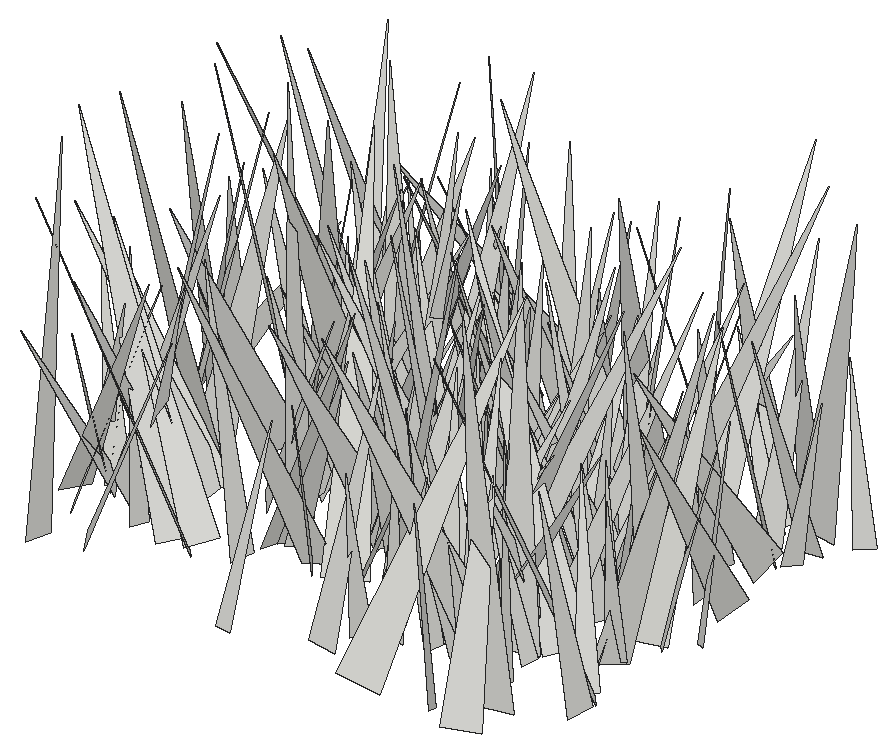
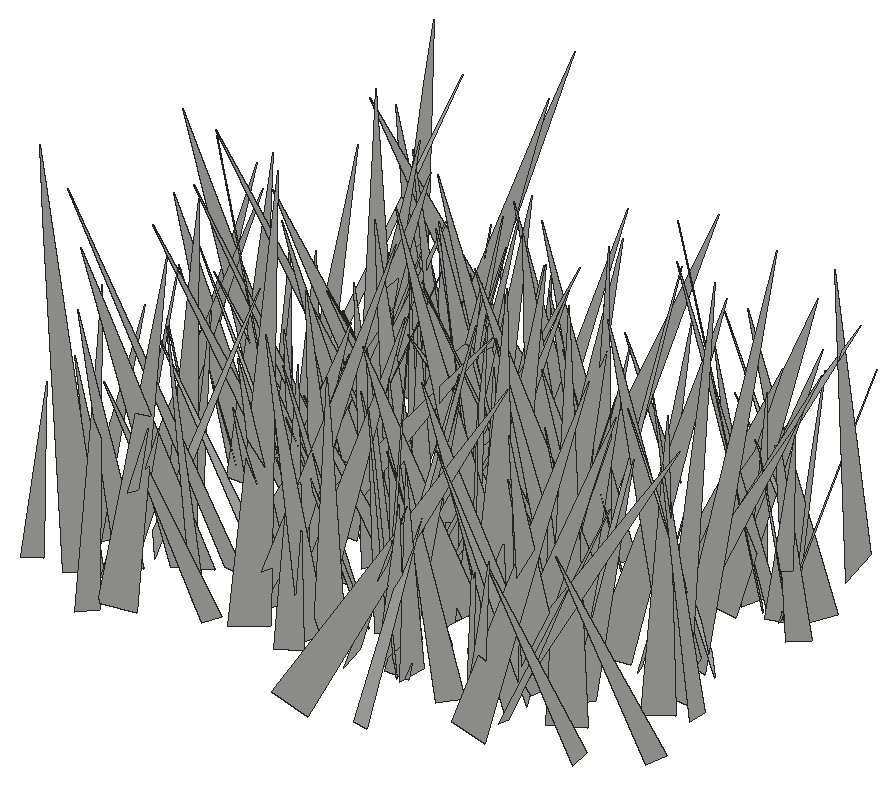
# SketchUp Ruby script. Lengths in inches.
U = 1.inch
M = Sketchup.active_model
def pt(a) = Geom::Point3d.new(a.map { |v| v * U })
def face(e, loops, mat)
  f = e.add_face(loops[0].map { |a| pt(a) })
  loops[1..].each { |l| e.add_face(l.map { |a| pt(a) }).erase! }
  f.material = f.back_material = mat if mat
  f
end
# faces: each face lists its corners as indices into pts; further lists are holes
def faces(e, pts, list, mat = nil) = list.each { |f| face(e, (f[0].is_a?(Array) ? f : [f]).map { |l| l.map { |i| pts[i] } }, mat) }
# xy, xz, yz: faces in a plane at the given z, y or x. An outline is a flat list of corners, or four numbers for a rectangle; further outlines are holes
def ring(l) = l.size == 4 ? [[l[0], l[1]], [l[2], l[1]], [l[2], l[3]], [l[0], l[3]]] : l.each_slice(2).to_a
def flat(e, list, mat, &to3) = list.each { |f| face(e, (f[0].is_a?(Array) ? f : [f]).map { |l| ring(l).map { |u, v| to3.(u, v) } }, mat) }
def xy(e, z, list, mat = nil) = flat(e, list, mat) { |x, y| [x, y, z] }
def xz(e, y, list, mat = nil) = flat(e, list, mat) { |x, z| [x, y, z] }
def yz(e, x, list, mat = nil) = flat(e, list, mat) { |y, z| [x, y, z] }
def lines(e, pts, list) = list.each { |a, b| e.add_line(pt(pts[a]), pt(pts[b])) }
# prism: a flat outline (further loops are holes) pulled along v
def prism(e, loops, v, mat = nil)
  f = face(e, loops, mat); d = Geom::Vector3d.new(v.map { |x| x * U })
  f.pushpull(f.normal.samedirection?(d) ? d.length : -d.length)
end
def box(e, o, s, mat = nil) = prism(e, [[o, [o[0] + s[0], o[1], o[2]], [o[0] + s[0], o[1] + s[1], o[2]], [o[0], o[1] + s[1], o[2]]]], [0, 0, s[2]], mat)
def at(x, y, z, deg = 0) = Geom::Transformation.translation(pt([x, y, z])) * Geom::Transformation.rotation(ORIGIN, Z_AXIS, deg.degrees)
def axes(o, x, y, z) = Geom::Transformation.new([*x, 0, *y, 0, *z, 0, *pt(o).to_a, 1])
def part(name) = M.definitions.add(name)
# library, detail: a bought-in or finely detailed component or shape, given as its bounding box
def library(name, o, s) = part(name).tap { |d| box(d.entities, o, s) }
def detail(e, o, s) = box(e.add_group.entities, o, s)
def put(e, d, t, mat = nil) = e.add_instance(d, t).tap { |i| i.material = mat if mat }
def group(e, t, mat = nil) = e.add_group.tap { |g| g.transformation = t; g.material = mat if mat }.entities
root = M.entities
c1 = part("fur_instance\#9")
p = [[0.8125,0,1.79],[0.67,-0.02,1.48],[0,-0.11,0],[0,0.11,0]]
faces(c1.entities,p,[[0,1,2,3]])
put(root,c1,axes([111.79,435.77,-27.1],[-2.18486,3.79279,1.02862],[3.92891,2.13324,0.47945],[0.08359,-1.13179,4.35074]))
put(root,c1,axes([111.93,431,-27.1],[-7.13651,-0.0123,2.39844],[-0.61978,7.28244,-1.80677],[2.31701,1.91008,6.90402]))
put(root,c1,axes([108.84,446.41,-27.1],[1.93678,-3.59499,0.72466],[-3.24209,-1.29543,2.2385],[1.71404,1.61186,3.41529]))
put(root,c1,axes([109.68,443.03,-27.1],[5.83398,1.13984,1.03884],[1.35175,-5.73614,-1.2974],[-0.74243,-1.48703,5.80098]))
put(root,c1,axes([111.72,435.73,-27.1],[-3.93384,-2.91751,0.42121],[-2.51987,3.69278,2.04402],[1.52955,-1.41982,4.45073]))
put(root,c1,axes([111.57,435.41,-27.1],[-2.88957,-1.62735,2.00469],[-2.2228,3.09866,-0.68855],[1.31385,1.66334,3.24403]))
put(root,c1,axes([110.3,436.45,-27.1],[2.04033,-4.0488,0.48109],[-4.03745,-1.93127,0.8697],[0.56854,0.81522,4.44965]))
put(root,c1,axes([110.85,443.78,-27.1],[3.52243,-4.25283,0.7835],[-4.27225,-3.57882,-0.21878],[-0.66956,0.46198,5.5178]))
put(root,c1,axes([112.21,440.22,-27.1],[-2.39726,-7.68863,1.50052],[-7.81274,2.46126,0.12966],[0.5725,1.39306,8.05265]))
put(root,c1,axes([111.07,442.56,-27.1],[-1.7083,-7.51191,1.45388],[-7.48357,1.95063,1.28533],[1.59333,1.10775,7.59572]))
put(root,c1,axes([111.57,439.72,-27.1],[4.49985,4.45709,1.03745],[4.28289,-4.6143,1.2473],[-1.61209,0.1822,6.20956]))
put(root,c1,axes([111.3,435.7,-27.1],[-2.16154,-4.08693,0.6496],[-3.73051,2.24163,1.68984],[1.79115,-0.26331,4.30345]))
put(root,c1,axes([114.72,437.71,-27.1],[-4.43376,3.47486,0.22998],[3.34427,4.14468,1.85019],[-0.97128,-1.59146,5.32068]))
put(root,c1,axes([114.79,437.59,-27.1],[-6.1435,0.43905,0.01492],[0.43419,6.03663,1.1429],[-0.06685,-1.14104,6.05221]))
put(root,c1,axes([116.16,446.22,-27.1],[-4.67528,-5.85921,0.505],[-5.43274,4.05599,-3.23694],[-2.25181,2.37953,6.76097]))
put(root,c1,axes([111.5,433.51,-27.1],[4.04394,2.43918,0.42992],[2.39305,-4.06014,0.52577],[-0.63852,0.23141,4.69325]))
put(root,c1,axes([115.94,434.08,-27.1],[-4.22364,6.9226,0.63988],[6.72709,3.88063,2.42031],[-1.75445,-1.78585,7.73974]))
put(root,c1,axes([111.04,448.03,-27.1],[4.1398,0.29454,0.02134],[0.28882,-4.10074,0.57065],[-0.06159,0.56772,4.11084]))
put(root,c1,axes([110.67,434.7,-27.1],[5.28357,-2.5058,0.04843],[-2.504,-5.27298,0.35108],[0.10676,0.33794,5.83712]))
put(root,c1,axes([113.52,444.75,-27.1],[-4.62696,1.13691,1.70574],[1.48296,4.76376,0.84751],[1.41525,-1.27471,4.68861]))
put(root,c1,axes([113.81,436.46,-27.1],[0.77993,-5.26102,0.56712],[-5.12867,-0.89269,-1.22806],[-1.30258,0.36472,5.1748]))
put(root,c1,axes([114.15,433.99,-27.1],[-5.02502,0.15502,0.9974],[-0.08895,4.97687,-1.22169],[1.00545,1.21508,4.87671]))
put(root,c1,axes([113.43,441.62,-27.1],[-3.15969,-2.10838,0.70871],[-1.88389,3.19122,1.09464],[1.18257,-0.54957,3.6374]))
put(root,c1,axes([116.91,433.47,-27.1],[-5.49378,-4.48735,0.1731],[-4.21573,5.05933,-2.64174],[-1.54724,2.14821,6.58325]))
put(root,c1,axes([116.55,444.95,-27.1],[-3.06653,-6.21678,2.70439],[-6.51984,1.89062,-3.04678],[-1.85842,3.62531,6.22648]))
put(root,c1,axes([112.43,440.375,-27.1],[-0.87926,6.56228,2.62812],[6.83144,1.46959,-1.38397],[1.81713,-2.34956,6.47466]))
put(root,c1,axes([114.84,447.625,-27.1],[-4.29176,-1.39668,0.34406],[-1.22552,4.11722,1.42648],[0.75311,-1.25938,4.28195]))
put(root,c1,axes([115.32,449.05,-27.1],[-0.75565,-7.24529,1.23648],[-7.25287,0.53359,-1.30585],[-1.19119,1.34729,7.16659]))
put(root,c1,axes([116.74,434.33,-27.1],[-3.94655,4.7323,0.06828],[4.56087,3.77904,1.70056],[-1.26405,-1.13963,5.92267]))
put(root,c1,axes([115.15,444.92,-27.1],[-6.13848,3.83375,0.83292],[3.60337,6.1212,-1.61832],[1.55148,0.95163,7.05405]))
put(root,c1,axes([112.15,435.48,-27.1],[3.4737,5.90005,1.74495],[6.11319,-3.08303,-1.74525],[0.69596,-2.36778,6.62052]))
put(root,c1,axes([113.13,435.06,-27.1],[5.7382,5.20942,1.87337],[5.41352,-5.84467,-0.3291],[-1.15821,-1.50876,7.74318]))
put(root,c1,axes([113.33,435.24,-27.1],[4.73571,-1.08461,0.9225],[-1.0987,-4.82145,-0.02851],[-0.90568,0.17765,4.85824]))
put(root,c1,axes([114.72,441.66,-27.1],[4.75153,-4.99406,0.9078],[-4.47168,-4.70683,-2.48828],[-2.40183,-1.11663,6.42854]))
put(root,c1,axes([112.9,446.44,-27.1],[1.80193,-7.44469,0.50754],[-7.36471,-1.69029,1.35351],[1.20089,0.80465,7.53912]))
put(root,c1,axes([116.74,440.5,-27.1],[-6.42891,-4.93695,1.78859],[-5.18873,6.40682,-0.96596],[0.80598,1.86616,8.04806]))
put(root,c1,axes([116.12,447.69,-27.1],[0.1057,3.9764,0.92499],[3.9126,-0.36287,1.11284],[-1.16573,-0.85739,3.81897]))
put(root,c1,axes([113.4,431.88,-27.1],[4.3525,2.53578,0.43229],[2.57081,-4.2585,-0.90411],[0.08934,-0.99816,4.9555]))
put(root,c1,axes([115.09,442.33,-27.1],[4.32331,2.64676,1.47041],[2.57631,-4.56233,0.63737],[-1.59061,-0.19566,5.02892]))
put(root,c1,axes([116.06,443.05,-27.1],[-2.49672,2.92464,0.96124],[2.97957,2.60694,-0.1927],[0.77439,-0.6012,3.84057]))
put(root,c1,axes([115.46,445.33,-27.1],[5.32876,3.34285,1.26399],[2.90072,-5.37113,1.97605],[-2.08763,1.0697,5.97207]))
put(root,c1,axes([116.81,442.59,-27.1],[-4.46885,1.59045,1.08144],[1.18804,4.43404,-1.61169],[1.51249,1.21632,4.46123]))
put(root,c1,axes([115.78,444.75,-27.1],[5.60712,-6.07402,0.33398],[-5.83929,-5.5015,-2.02021],[-1.70529,-1.13347,8.01575]))
put(root,c1,axes([114.31,443.875,-27.1],[6.51578,-0.90085,0.09034],[-0.89347,-6.50413,-0.41604],[-0.1463,-0.39981,6.56459]))
put(root,c1,axes([117.02,443.31,-27.1],[-4.18199,-2.55213,0.91155],[-1.98836,4.02848,2.15666],[1.84139,-1.44616,4.39901]))
put(root,c1,axes([118.53,434.42,-27.1],[-5.56537,0.35389,1.01892],[0.25962,5.63719,-0.53984],[1.04691,0.48332,5.55042]))
put(root,c1,axes([118.64,437.53,-27.1],[-8.04005,-0.21045,2.18635],[-0.63833,8.16213,-1.56173],[2.10165,1.67397,7.88972]))
put(root,c1,axes([117.86,439.8125,-27.1],[-4.50462,1.14541,2.32905],[1.86637,4.67145,1.31236],[1.80364,-1.97324,4.45884]))
put(root,c1,axes([116.33,444.74,-27.1],[-3.15581,4.82371,2.67558],[4.59437,4.00448,-1.80054],[3.05265,-1.04019,5.47589]))
put(root,c1,axes([118.45,443.82,-27.1],[5.58768,-4.04107,3.86555],[-4.58295,-6.44048,-0.10822],[-3.20457,2.16447,6.89498]))
put(root,c1,axes([116.71,447.23,-27.1],[-2.8265,-4.26887,1.57231],[-3.66111,3.23328,2.19698],[2.70032,-0.08465,4.62446]))
put(root,c1,axes([117.77,444.52,-27.1],[1.5026,-5.2869,1.47769],[-5.48951,-1.44343,0.41772],[0.01326,1.53554,5.48039]))
put(root,c1,axes([116.67,438.11,-27.1],[3.8282,2.91024,0.83789],[3.01788,-3.55309,-1.44728],[0.25298,-1.65308,4.58585]))
put(root,c1,axes([116.37,440.34,-27.1],[6.24865,-3.61776,1.18124],[-3.80474,-5.99015,1.78079],[-0.08657,2.13519,6.99733]))
put(root,c1,axes([118.68,451,-27.1],[-3.43446,-5.67079,0.15135],[-5.3482,3.29577,2.1239],[1.89143,-0.97791,6.28032]))
put(root,c1,axes([119.51,447.02,-27.1],[-4.59387,1.36569,1.34916],[1.20913,4.77619,-0.71765],[1.49109,0.33451,4.73854]))
put(root,c1,axes([117.33,447.59,-27.1],[2.31038,-4.41979,0.71264],[-4.3801,-2.06578,1.38834],[0.92579,1.25629,4.79008]))
put(root,c1,axes([120.58,446.91,-27.1],[-3.8761,2.85036,0.12124],[2.83481,3.87102,-0.37744],[0.32105,0.23257,4.79648]))
put(root,c1,axes([121.63,451.375,-27.1],[2.28844,-6.77562,0.58153],[-5.77223,-2.2597,-3.61376],[-3.59563,-0.68473,6.17144]))
put(root,c1,axes([120.97,435.77,-27.1],[0.32689,-6.93131,1.01824],[-6.72809,-0.59471,-1.88835],[-1.95261,0.88881,6.67713]))
put(root,c1,axes([119.48,436.3,-27.1],[4.39596,-0.31282,2.17467],[-1.10489,-4.51925,1.5834],[-1.89902,1.90528,4.11281]))
put(root,c1,axes([120.54,441,-27.1],[-3.35147,5.54659,2.9979],[6.27053,3.28643,0.92965],[0.65767,-3.06906,6.41348]))
put(root,c1,axes([121.12,446.57,-27.1],[-6.29577,-3.22015,2.48262],[-3.79064,6.30377,-1.43636],[1.47099,2.46225,6.92409]))
put(root,c1,axes([121.97,447.4,-27.1],[-4.83845,-0.36416,0.05457],[-0.36621,4.6838,-1.21411],[-0.03844,1.21473,4.69778]))
put(root,c1,axes([119.9375,447.37,-27.1],[-0.22883,-5.12281,0.23524],[-5.12454,0.23734,0.18366],[0.19416,0.22665,5.12463]))
put(root,c1,axes([120.32,447.08,-27.1],[3.4021,4.35261,1.87369],[4.47593,-3.70904,0.48912],[-1.55627,-1.15238,5.50275]))
put(root,c1,axes([117.35,440.14,-27.1],[4.17015,5.48726,0.52169],[5.30168,-3.81404,-2.26221],[1.50809,-1.76505,6.51019]))
put(root,c1,axes([120.72,442.78,-27.1],[-6.29891,4.40553,1.36932],[3.82289,6.28157,-2.62437],[2.58248,1.44677,7.22479]))
put(root,c1,axes([118.68,440.96,-27.1],[2.58495,3.56171,0.23056],[3.43761,-2.40789,-1.34382],[0.96012,-0.96809,4.1907]))
put(root,c1,axes([119.54,440.2,-27.1],[4.26328,-1.39926,0.74192],[-1.39292,-4.32659,-0.15583],[-0.75375,0.08115,4.48433]))
put(root,c1,axes([119.57,444.69,-27.1],[3.16954,2.48643,0.53995],[2.54162,-3.13416,-0.48689],[-0.1185,-0.71733,3.99891]))
put(root,c1,axes([120.68,442.48,-27.1],[5.22033,-0.21574,2.13038],[0.1303,-5.5713,-0.88347],[-2.13731,-0.86658,5.14955]))
put(root,c1,axes([122.38,435.47,-27.1],[-3.14428,7.71271,0.49149],[7.72648,3.12546,0.38342],[-0.17032,-0.59964,8.32018]))
put(root,c1,axes([122.85,439.9,-27.1],[-6.22259,1.31552,1.1088],[1.51746,6.15727,1.21077],[0.81078,-1.42761,6.24382]))
put(root,c1,axes([119.25,436.41,-27.1],[4.36325,-2.68491,0.18726],[-2.69098,-4.34538,0.39756],[0.04948,0.43666,5.1077]))
put(root,c1,axes([121.28,429.87,-27.1],[1.03899,3.82207,0.22987],[3.79032,-1.06041,0.49963],[-0.54276,-0.08876,3.92914]))
put(root,c1,axes([118.87,436.01,-27.1],[6.16535,-1.94029,0.16764],[-1.94054,-6.16752,-0.01601],[-0.16472,0.03505,6.46343]))
put(root,c1,axes([122.63,443.95,-27.1],[-6.25427,-0.78477,1.30734],[-0.71032,6.38344,0.43371],[1.34924,-0.27711,6.28838]))
put(root,c1,axes([118.12,443.25,-27.1],[8.10386,-2.02713,0.06413],[-2.02706,-8.10412,-0.01624],[-0.06615,-0.00019,8.35354]))
put(root,c1,axes([120.83,435.52,-27.1],[-2.98653,-2.99705,1.42564],[-2.58075,3.30304,1.53746],[2.08674,-0.20437,3.94181]))
put(root,c1,axes([121.02,438.68,-27.1],[4.46685,2.95329,0.59597],[2.75098,-4.43263,1.34675],[-1.2285,0.81223,5.18275]))
put(root,c1,axes([121.8,438.78,-27.1],[6.11084,-2.63091,1.80363],[-1.49433,-5.80472,-3.40432],[-2.81811,-2.62692,5.71618]))
put(root,c1,axes([121.27,445.14,-27.1],[3.01124,-3.84874,1.35887],[-4.04465,-3.04041,0.35153],[-0.54781,1.29229,4.87409]))
put(root,c1,axes([124.53,439.91,-27.1],[-6.85321,0.30824,0.48855],[0.41589,6.6696,1.62593],[0.40091,-1.64973,6.66467]))
put(root,c1,axes([123.75,440.92,-27.1],[-4.70083,-1.74871,0.0814],[-1.70109,4.61801,0.97093],[0.41342,-0.88228,4.92068]))
put(root,c1,axes([123.51,446.72,-27.1],[-0.65155,5.99766,1.58433],[6.18323,0.49957,0.65163],[-0.49968,-1.63861,5.99765]))
put(root,c1,axes([122.21,438.33,-27.1],[6.62959,-1.41825,2.66639],[-1.99694,-6.88369,1.30369],[-2.26567,1.91728,6.65307]))
put(root,c1,axes([122.86,438.14,-27.1],[2.86729,-4.50295,0.62999],[-4.43501,-2.93396,-0.78577],[-1.00209,0.10064,5.2802]))
put(root,c1,axes([122.16,440.4375,-27.1],[1.97582,-3.11414,0.08334],[-3.10691,-1.9626,0.3224],[0.22782,0.24287,3.67393]))
put(root,c1,axes([124.13,436.48,-27.1],[-7.73799,2.57835,1.8542],[1.9672,7.72518,-2.53263],[2.4932,1.90688,7.75308]))
put(root,c1,axes([125.91,437.43,-27.1],[-7.81157,-0.92448,1.21309],[-1.13809,7.74743,-1.42443],[1.01538,1.5715,7.73604]))
put(root,c1,axes([124.1,437.6875,-27.1],[1.75802,-6.33898,1.96931],[-6.51413,-2.03906,-0.74828],[-1.27556,1.67662,6.53555]))
put(root,c1,axes([123.1,435.31,-27.1],[4.98815,3.01806,0.37753],[2.59556,-4.60182,2.49383],[-1.58564,1.9615,5.26983]))
put(root,c1,axes([122.125,445.13,-27.1],[0.90872,-5.0896,0.45336],[-4.90772,-0.74115,1.51668],[1.42262,0.69427,4.94262]))
put(root,c1,axes([124.6,446.9375,-27.1],[2.95346,-5.37759,1.21149],[-5.08452,-3.18852,-1.75785],[-2.12927,0.1548,5.87804]))
put(root,c1,axes([128.625,441.75,-27.1],[-5.00631,-5.98003,0.73957],[-5.22244,3.82659,-4.41068],[-3.00563,3.31169,6.43193]))
put(root,c1,axes([126.08,437.46,-27.1],[-6.2227,2.39174,0.32304],[2.36421,6.22042,-0.51348],[0.48507,0.36431,6.64671]))
put(root,c1,axes([126.85,446.18,-27.1],[-8.04315,1.60644,1.39343],[1.83623,7.99603,1.38066],[1.07265,-1.64234,8.08496]))
put(root,c1,axes([123.91,442.05,-27.1],[3.88682,0.49651,1.01606],[0.42112,-4.01087,0.34905],[-1.04955,0.22945,3.90283]))
put(root,c1,axes([123.05,445.28,-27.1],[2.48404,3.35431,0.63876],[3.34518,-2.23213,-1.28736],[0.685,-1.26336,3.97047]))
put(root,c1,axes([127.67,435.57,-27.1],[-6.96753,-1.64469,0.65915],[-1.76863,6.61713,-2.18437],[0.10697,2.27915,6.81763]))
put(root,c1,axes([125.1875,443.42,-27.1],[1.99951,5.4557,0.6063],[5.41529,-2.06607,0.73224],[-0.89823,-0.31139,5.76424]))
put(root,c1,axes([123.96,447.08,-27.1],[5.74343,-0.59024,1.12729],[-0.57342,-5.85294,-0.14303],[-1.13593,-0.02976,5.77191]))
put(root,c1,axes([123.78,442.05,-27.1],[-0.24087,4.17753,0.95098],[3.88217,0.61574,-1.72155],[1.81241,-0.76371,3.81393]))
put(root,c1,axes([124.8,431.11,-27.1],[0.44242,5.64748,1.29703],[5.78226,-0.34572,-0.46699],[0.37666,-1.32609,5.6455]))
put(root,c1,axes([124.14,448.28,-27.1],[1.58205,-4.94043,0.08132],[-4.90313,-1.55912,0.66773],[0.6114,0.28046,5.1444]))
put(root,c1,axes([125.51,434,-27.1],[-5.11664,3.91829,0.85035],[3.38571,4.96082,-2.48663],[2.14782,1.51438,5.94556]))
put(root,c1,axes([125.46,432.53,-27.1],[2.03457,-2.99845,1.01926],[-3.06758,-2.16697,-0.25148],[-0.78708,0.69471,3.61482]))
put(root,c1,axes([124.48,440.99,-27.1],[4.31409,-4.88001,1.43702],[-5.06352,-4.30068,0.59646],[-0.49016,1.47666,6.48614]))
put(root,c1,axes([125.49,441.46,-27.1],[-4.36102,2.95909,2.58691],[3.11538,4.95832,-0.41976],[2.39639,-1.06094,5.25343]))
put(root,c1,axes([128.03,433.61,-27.1],[-6.43885,-0.2283,0.73687],[-0.34147,6.39798,-1.00159],[0.69173,1.03328,6.36457]))
put(root,c1,axes([123.48,439.1875,-27.1],[7.4678,0.08394,0.57516],[0.2355,-7.21321,-2.00499],[-0.53141,-2.01703,7.1941]))
put(root,c1,axes([126.61,437.625,-27.1],[-4.17339,1.81444,1.20525],[1.74242,4.34394,-0.50613],[1.30721,0.0026,4.52253]))
put(root,c1,axes([126.13,432.95,-27.1],[6.62272,2.03005,2.53711],[1.31072,-6.93962,2.13125],[-2.97322,1.46257,6.59085]))
put(root,c1,axes([124.73,439.93,-27.1],[0.74077,3.76285,1.03817],[3.63302,-0.27816,-1.5841],[1.42759,-1.24465,3.49262]))
put(root,c1,axes([126.15,443.51,-27.1],[-1.18817,5.57554,2.26119],[5.96275,1.39894,-0.31626],[0.80332,-2.13721,5.69196]))
put(root,c1,axes([126.49,433.08,-27.1],[0.16475,-3.83195,1.51207],[-4.1166,-0.0965,0.20397],[0.15418,1.51796,3.83006]))
put(root,c1,axes([129.53,438.83,-27.1],[-6.43064,-2.17008,0.24743],[-2.17262,6.27662,-1.4168],[-0.22404,1.42068,6.6374]))
put(root,c1,axes([126.78,440.1,-27.1],[2.27684,-3.73592,1.683],[-3.94498,-2.51908,-0.25488],[-1.10756,1.29258,4.36763]))
put(root,c1,axes([129.45,433.69,-27.1],[-0.93338,-7.69941,2.7531],[-7.87622,0.10215,-2.38461],[-2.19672,2.90522,7.38009]))
put(root,c1,axes([126.33,432.98,-27.1],[2.59266,-2.6088,0.97622],[-2.78019,-2.50569,0.68761],[-0.17141,1.18171,3.61316]))
put(root,c1,axes([126.36,445.94,-27.1],[-1.839,3.01934,1.93742],[3.07994,2.44517,-0.88715],[1.83955,-1.07548,3.42218]))
put(root,c1,axes([128.46,444,-27.1],[-4.34148,-1.68145,0.56308],[-1.64517,4.37512,0.38015],[0.66161,-0.1544,4.64018]))
put(root,c1,axes([128.1,434.09,-27.1],[-0.91047,5.0165,1.03079],[5.11456,0.83694,0.44447],[-0.2628,-1.09133,5.07905]))
put(root,c1,axes([127.39,437.1,-27.1],[4.14484,0.5886,1.74948],[0.68446,-4.48393,-0.11303],[-1.71425,-0.36717,4.1849]))
put(root,c1,axes([128.9,443.1875,-27.1],[0.42359,6.38348,0.10104],[6.1795,-0.43539,1.60081],[-1.60398,0.00839,6.194]))
put(root,c1,axes([126.3,447.83,-27.1],[7.64117,-3.1953,0.94942],[-2.87226,-7.51641,-2.18001],[-1.69158,-1.67105,7.9903]))
put(root,c1,axes([125.59,437.76,-27.1],[2.92691,3.10527,0.26779],[2.82947,-2.4932,-2.01476],[1.3071,-1.55642,3.76168]))
put(root,c1,axes([128.03,440.64,-27.1],[0.49777,-7.47829,0.86543],[-7.52286,-0.52678,-0.22508],[-0.28353,0.84808,7.49146]))
put(root,c1,axes([129.28,434.875,-27.1],[-7.73279,0.49202,2.83462],[1.75633,7.24586,3.53356],[2.27869,-3.91518,6.89581]))
put(root,c1,axes([130.17,441.54,-27.1],[0.21984,-5.04241,1.33274],[-4.72838,-0.75562,-2.0789],[-2.20101,1.11963,4.59917]))
put(root,c1,axes([126.64,436.78,-27.1],[0.2906,4.64928,0.9365],[4.41539,0.07727,-1.75374],[1.73123,-0.9775,4.31562]))
put(root,c1,axes([130.64,438.02,-27.1],[-3.35511,-5.27651,0.83113],[-5.27558,3.11951,-1.49198],[-0.83701,1.48869,6.07225]))
put(root,c1,axes([128.56,440.55,-27.1],[-0.5351,4.97369,0.08314],[4.96853,0.53845,-0.2337],[0.24128,-0.05757,4.99693]))
put(root,c1,axes([127.36,439.38,-27.1],[0.34617,6.42334,1.62872],[6.51894,-0.03728,-1.2385],[1.18972,-1.66468,6.31231]))
put(root,c1,axes([131.8125,436.34,-27.1],[-7.18183,4.15456,0.03319],[4.14203,7.15453,0.70461],[-0.3242,-0.62648,8.26695]))
put(root,c1,axes([131.4,438.75,-27.1],[0.1109,6.16383,0.84068],[5.38265,-0.51661,3.07768],[-3.11876,-0.67243,5.34163]))
put(root,c1,axes([130.74,430.02,-27.1],[-5.03149,-1.83162,1.20846],[-2.18082,4.50919,-2.24552],[0.24343,2.5384,4.86091]))
put(root,c1,axes([129.83,440.49,-27.1],[-3.46593,0.7925,0.89611],[1.04093,3.35143,1.06213],[0.58952,-1.25841,3.39303]))
put(root,c1,axes([128.09,437.3125,-27.1],[4.34491,0.59069,1.09524],[0.90101,-4.23706,-1.28924],[-0.85828,-1.45776,4.19106]))
put(root,c1,axes([127.49,429.8125,-27.1],[-1.94232,7.80928,1.11049],[7.41359,2.19794,-2.48968],[2.69386,-0.41817,7.65238]))
put(root,c1,axes([129.58,446.77,-27.1],[-5.36603,-1.88935,2.74168],[-2.67241,5.54565,-1.40882],[1.98613,2.35731,5.51173]))
put(root,c1,axes([129.06,441.46,-27.1],[0.06663,3.86387,1.64805],[4.18879,0.06273,-0.31643],[0.31563,-1.6482,3.85147]))
put(root,c1,axes([128.0625,436.15,-27.1],[6.72656,-0.08852,1.07497],[-0.40385,-6.50233,1.99163],[-1.00015,2.03024,6.42556]))
put(root,c1,axes([131.33,434.8125,-27.1],[-3.91396,0.19988,0.40503],[0.19284,3.93443,-0.07818],[0.40843,0.05784,3.91828]))
put(root,c1,axes([127.61,448.34,-27.1],[1.13497,4.33314,1.68645],[4.04549,-0.06445,-2.557],[2.29221,-2.03177,3.67778]))
put(root,c1,axes([130.5,435.17,-27.1],[1.64686,-6.77743,3.62945],[-7.62252,-1.92308,-0.13234],[-1.0018,3.49096,6.97339]))
put(root,c1,axes([132.68,445.33,-27.1],[-5.08452,-4.09315,0.88657],[-4.17476,4.84247,-1.58557],[-0.33349,1.78573,6.33184]))
put(root,c1,axes([131.56,433.22,-27.1],[-4.31752,-0.25034,0.73123],[-0.52227,4.00392,-1.71296],[0.56974,1.77322,3.97108]))
put(root,c1,axes([130.98,436.93,-27.1],[-4.32918,-1.79601,0.73607],[-1.48596,4.22424,1.56749],[1.24875,-1.19977,4.41706]))
put(root,c1,axes([128.19,436.72,-27.1],[3.14457,7.68443,0.45621],[7.56933,-2.99688,-1.69436],[1.40136,-1.05601,8.12822]))
put(root,c1,axes([130.8125,449.74,-27.1],[2.01145,-6.31603,1.30369],[-6.40118,-2.12156,-0.40211],[-0.78536,1.11557,6.61638]))
put(root,c1,axes([132.23,448.24,-27.1],[-2.23276,3.13779,0.67741],[3.20125,2.1153,0.75324],[-0.23799,-0.9847,3.77672]))
put(root,c1,axes([130.43,442.67,-27.1],[4.1336,3.03674,0.5342],[2.87698,-4.11997,1.15876],[-1.10914,0.6308,4.99657]))
put(root,c1,axes([132.42,447.4,-27.1],[-3.36159,2.04077,0.19725],[2.04893,3.35754,0.1809],[0.07444,-0.25709,3.9284]))
put(root,c1,axes([130.5,445.8125,-27.1],[-1.86477,7.56726,1.18834],[7.49142,2.05683,-1.34204],[1.5982,-0.81177,7.67722]))
put(root,c1,axes([128.96,435.21,-27.1],[4.72114,-1.50275,0.05764],[-1.46013,-4.53503,1.361],[0.36002,1.31378,4.76394]))
put(root,c1,axes([131.54,430.97,-27.1],[2.89571,-2.97183,2.13904],[-3.49598,-3.05481,0.48854],[-1.08874,1.90494,4.12046]))
put(root,c1,axes([132.45,431.35,-27.1],[0.36283,-7.33481,3.26148],[-7.98321,-0.67122,-0.62142],[-0.83968,3.21222,7.31744]))
put(root,c1,axes([129.13,445.09,-27.1],[3.76818,7.24013,0.96766],[7.17608,-3.46602,-2.01138],[1.36373,-1.76699,7.91031]))
put(root,c1,axes([132.47,429.47,-27.1],[-2.78795,6.31949,0.96814],[6.36227,2.84625,-0.25738],[0.62828,-0.78026,6.90234]))
put(root,c1,axes([130.36,437.72,-27.1],[2.81698,6.47491,0.35167],[6.46114,-2.77024,-0.75032],[0.54938,-0.62035,7.02117]))
put(root,c1,axes([130.69,439.76,-27.1],[1.99959,6.47326,0.24716],[6.43471,-1.95494,-0.85747],[0.74746,-0.48749,6.72058]))
put(root,c1,axes([132.1,438.68,-27.1],[5.36611,5.59511,2.05394],[5.5109,-5.71038,1.15783],[-2.27022,-0.63666,7.66549]))
put(root,c1,axes([130.46,439.95,-27.1],[4.29759,3.17988,0.45483],[3.21134,-4.23507,-0.73441],[0.07624,-0.86047,5.29543]))
put(root,c1,axes([134.57,434.45,-27.1],[-5.605,-5.08718,0.25266],[-5.09303,5.60246,-0.18084],[0.06544,0.30374,7.56721]))
put(root,c1,axes([132.5,446.96,-27.1],[-0.07417,5.83715,1.21265],[5.95855,0.11247,-0.17697],[0.19614,-1.2097,5.83493]))
put(root,c1,axes([131.5,450.6,-27.1],[5.7747,-1.11479,0.95698],[-0.77258,-5.60537,-1.86777],[-1.24967,-1.68603,5.57685]))
put(root,c1,axes([133.22,437.3,-27.1],[3.01506,-0.72225,2.0256],[-1.00024,-3.559,0.21985],[-1.90373,0.72607,3.09256]))
put(root,c1,axes([133,439.83,-27.1],[0.27233,-6.25887,1.87066],[-6.53155,-0.29195,-0.02597],[-0.1084,1.8677,6.26474]))
put(root,c1,axes([133.22,442.27,-27.1],[3.59976,0.06174,1.80471],[0.19659,-4.01441,-0.2548],[-1.79504,-0.31584,3.59126]))
put(root,c1,axes([133.38,446.1,-27.1],[-3.17607,-4.40082,1.193],[-4.40846,3.33508,0.56622],[1.16445,0.62283,5.3976]))
put(root,c1,axes([132.36,444.23,-27.1],[5.38586,-3.00561,1.16634],[-2.8404,-5.49795,-1.05176],[-1.52519,-0.37466,6.07741]))
put(root,c1,axes([133.42,435.96,-27.1],[3.56764,3.88458,0.34534],[3.52617,-3.41301,1.96335],[-1.66594,1.09483,4.89523]))
put(root,c1,axes([134.27,434.41,-27.1],[-2.51117,3.39602,0.58609],[3.43959,2.51478,0.1658],[0.21361,-0.57041,4.22035]))
put(root,c1,axes([133.65,445.54,-27.1],[5.96418,-2.86813,1.57613],[-1.66285,-5.47776,-3.67572],[-2.81874,-2.83722,5.50334]))
put(root,c1,axes([134.23,447.26,-27.1],[-0.19346,-4.85951,0.89963],[-4.92735,0.1202,-0.41034],[-0.38132,0.91231,4.84602]))
put(root,c1,axes([133.66,436.8125,-27.1],[1.81522,-3.21568,0.8696],[-3.29805,-1.87418,-0.04607],[-0.46866,0.73395,3.69235]))
put(root,c1,axes([133.78,438.57,-27.1],[-3.09006,5.24053,1.65653],[5.13422,3.43055,-1.27548],[1.9614,-0.72379,5.94851]))
put(root,c1,axes([135.01,433.1,-27.1],[4.20178,-1.75309,2.00996],[-1.5081,-4.65512,-0.90755],[-2.19975,-0.15714,4.46146]))
put(root,c1,axes([135.3,439.62,-27.1],[2.28996,3.33239,0.84649],[3.03653,-2.43723,1.38011],[-1.61271,0.14282,3.80053]))
put(root,c1,axes([133.64,436.53,-27.1],[6.60662,-2.19065,2.41659],[-2.83754,-6.55209,1.81792],[-1.6085,2.56075,6.71874]))
put(root,c1,axes([134.22,446.19,-27.1],[3.08181,-1.73974,0.98019],[-1.88437,-3.1302,0.36886],[-0.66077,0.81254,3.51969]))
put(root,c1,axes([134.17,438.76,-27.1],[2.95956,2.83712,0.75066],[2.89518,-2.997,-0.08741],[-0.48027,-0.58351,4.09885]))
put(root,c1,axes([134.63,442.34,-27.1],[5.34512,-3.23236,0.64666],[-2.65449,-4.95104,-2.80671],[-1.95449,-2.11559,5.5804]))
put(root,c1,axes([135.48,448.77,-27.1],[-2.21806,2.84038,1.31516],[3.07662,2.27502,0.2754],[0.57601,-1.21396,3.59328]))
put(root,c1,axes([133.36,448.5,-27.1],[1.45469,-7.67033,1.86376],[-7.74266,-1.0178,1.85445],[1.53584,2.13396,7.5836]))
